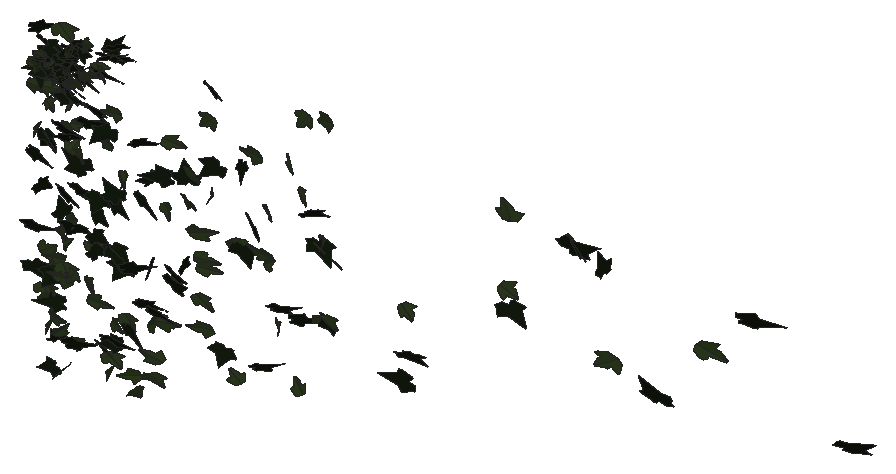
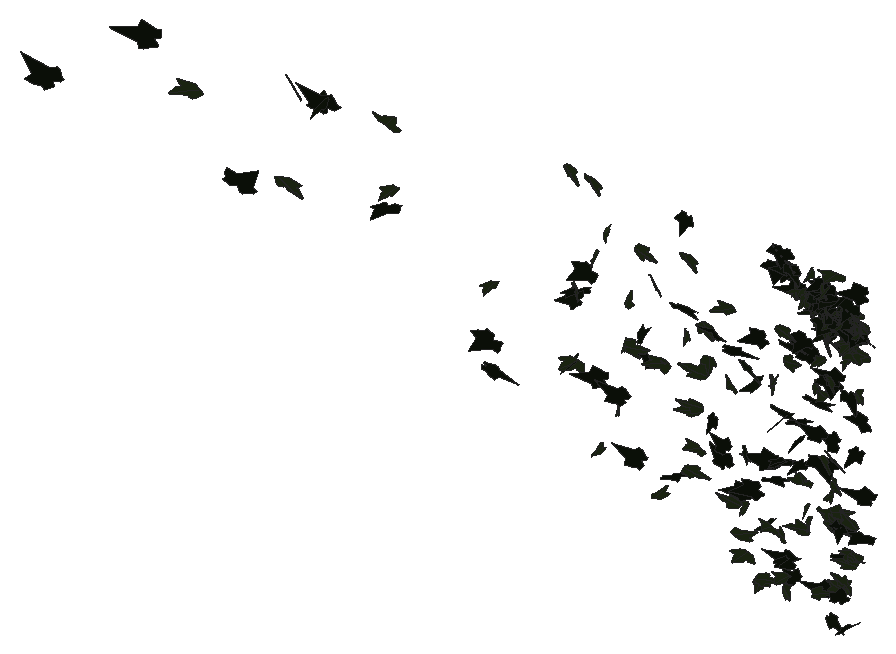
# SketchUp Ruby script. Lengths in millimetres.
U = 1.mm
M = Sketchup.active_model
def pt(a) = Geom::Point3d.new(a.map { |v| v * U })
def face(e, loops, mat)
  f = e.add_face(loops[0].map { |a| pt(a) })
  loops[1..].each { |l| e.add_face(l.map { |a| pt(a) }).erase! }
  f.material = f.back_material = mat if mat
  f
end
# faces: each face lists its corners as indices into pts; further lists are holes
def faces(e, pts, list, mat = nil) = list.each { |f| face(e, (f[0].is_a?(Array) ? f : [f]).map { |l| l.map { |i| pts[i] } }, mat) }
# xy, xz, yz: faces in a plane at the given z, y or x. An outline is a flat list of corners, or four numbers for a rectangle; further outlines are holes
def ring(l) = l.size == 4 ? [[l[0], l[1]], [l[2], l[1]], [l[2], l[3]], [l[0], l[3]]] : l.each_slice(2).to_a
def flat(e, list, mat, &to3) = list.each { |f| face(e, (f[0].is_a?(Array) ? f : [f]).map { |l| ring(l).map { |u, v| to3.(u, v) } }, mat) }
def xy(e, z, list, mat = nil) = flat(e, list, mat) { |x, y| [x, y, z] }
def xz(e, y, list, mat = nil) = flat(e, list, mat) { |x, z| [x, y, z] }
def yz(e, x, list, mat = nil) = flat(e, list, mat) { |y, z| [x, y, z] }
def lines(e, pts, list) = list.each { |a, b| e.add_line(pt(pts[a]), pt(pts[b])) }
# prism: a flat outline (further loops are holes) pulled along v
def prism(e, loops, v, mat = nil)
  f = face(e, loops, mat); d = Geom::Vector3d.new(v.map { |x| x * U })
  f.pushpull(f.normal.samedirection?(d) ? d.length : -d.length)
end
def box(e, o, s, mat = nil) = prism(e, [[o, [o[0] + s[0], o[1], o[2]], [o[0] + s[0], o[1] + s[1], o[2]], [o[0], o[1] + s[1], o[2]]]], [0, 0, s[2]], mat)
def at(x, y, z, deg = 0) = Geom::Transformation.translation(pt([x, y, z])) * Geom::Transformation.rotation(ORIGIN, Z_AXIS, deg.degrees)
def axes(o, x, y, z) = Geom::Transformation.new([*x, 0, *y, 0, *z, 0, *pt(o).to_a, 1])
def part(name) = M.definitions.add(name)
# library, detail: a bought-in or finely detailed component or shape, given as its bounding box
def library(name, o, s) = part(name).tap { |d| box(d.entities, o, s) }
def detail(e, o, s) = box(e.add_group.entities, o, s)
def put(e, d, t, mat = nil) = e.add_instance(d, t).tap { |i| i.material = mat if mat }
def group(e, t, mat = nil) = e.add_group.tap { |g| g.transformation = t; g.material = mat if mat }.entities
root = M.entities
M.materials.add("efeu1").color = [18, 25, 13]
M.materials.add("efeu2").color = [43, 57, 29]
c1 = part("ivyleaf_9")
p = [[39.1,54.8,31.7],[34.5,51.8,30.2],[-5.3,25.2,17.3],[-17.9,28.3,20.9],[-21.6,21.7,17],[-20.2,4.3,5.3],
  [-22.9,-0.3,2.5],[-17.1,-4,-0.6],[-2,-2.1,-1.2],[-0.7,-15.4,-10.1],[16.6,-22.3,-16.7],[21.1,-15.1,-12.5],
  [32.7,-10.7,-11],[46.1,-1.8,-6.6],[30.8,11.2,3.8]]
faces(c1.entities,p,[[0,1,2,3,4,5,6,7,8,9,10,11,12,13,14]],"efeu1")
c2 = part("ivyleaf_10")
p = [[0,12.8,-0.8],[-1.5,51.3,-10.9],[-4.9,51,-11.6],[-13.6,26.5,-7.3],[-13.2,15.9,-4.6],[-21.1,19.3,-7.2],
  [-29.5,16.3,-8.3],[-29.2,8.3,-6.2],[-19.7,-9.8,0.5],[-7.6,-13,4],[1,-12.2,5.8],[-0.4,51.1,-11.1],
  [-1.5,51.1,-10.9],[1,-12.4,5.9],[16.9,-12.4,3.5],[35.1,9.1,-5.1],[35,12.9,-6.1],[20.5,16.4,-4.9],
  [15.8,15,-3.8],[15.3,27.6,-7.1],[12.8,31.3,-7.8]]
faces(c2.entities,p,[[0,1,2,3,4,5,6,7,8,9,10],[11,12,0,13,14,15,16,17,18,19,20]],"efeu2")
put(root,c1,axes([2770.4,996,647.1],[-0.43445,-0.41546,-0.67356],[0.58698,0.59889,-0.47393],[1.38708,-0.38357,-0.01041]))
put(root,c1,axes([2810.1,994.4,1431.9],[-1.27919,0.3991,0.09668],[-0.21391,-0.00043,-0.77958],[-0.75169,-0.67905,0.05732]))
put(root,c1,axes([2754.7,988,793.5],[0.65605,-0.1407,0.72585],[1.38247,-0.08487,-0.36142],[0.26236,0.79905,0.08942]))
put(root,c2,axes([2790.1,1023.7,1355.9],[1.07633,0.46383,-0.26625],[-0.4274,-0.14573,-0.73088],[-0.92378,0.60785,0.02794]))
put(root,c2,axes([2787.5,994.3,1427.6],[0.14869,0.78127,-0.03035],[-0.07273,-0.02665,-0.78437],[-1.48625,0.07947,0.03535]))
put(root,c2,axes([2792.4,997.3,1191.2],[0.28219,-0.75376,0.3272],[0.17611,-0.31505,-0.76771],[1.55394,0.17259,0.02758]))
put(root,c2,axes([2766.3,990.4,1346.9],[-0.16001,-0.05129,-0.78981],[1.38192,-0.32107,-0.05644],[-0.59945,-0.72649,0.0807]))
put(root,c1,axes([2795.2,996.2,965.3],[0.00384,-0.03525,-0.90722],[-0.71675,0.82546,-0.03291],[1.57226,0.37639,-0.01279]))
put(root,c2,axes([2788.9,993.1,1443.8],[0.95422,0.59568,0.11552],[0.13095,0.09307,-0.77857],[-1.14738,0.50602,0.00721]))
put(root,c1,axes([2792.6,992.2,1426.2],[1.13022,0.51418,-0.05023],[-0.05686,-0.04222,-0.78542],[-0.9816,0.59447,-0.01234]))
put(root,c1,axes([2767.1,988.9,1088.7],[0.30092,0.00107,-0.85529],[1.60853,0.13322,0.15641],[0.24969,-0.85952,0.02318]))
put(root,c2,axes([2793,983.8,1457.4],[-1.08334,-0.41986,-0.41689],[0.75174,0.16106,-0.70152],[0.83841,-0.68693,0.09033]))
put(root,c2,axes([2807,987.4,1445.8],[0.11013,-0.79891,-0.00714],[-0.00685,0.00689,-0.801],[1.52054,0.05789,-0.00309]))
put(root,c1,axes([2781.9,983.3,1575.3],[0.73988,0.19969,0.83467],[1.34298,0.44717,-0.43565],[-0.92968,0.80489,0.03495]))
put(root,c2,axes([2802.5,994.8,1447.7],[1.4992,0.02043,-0.01835],[-0.03497,0.00059,-0.78799],[-0.03885,0.78794,0.00107]))
put(root,c2,axes([2802.8,991.4,1449.2],[-1.33687,-0.27071,-0.23913],[0.49196,-0.01151,-0.74628],[0.48015,-0.74193,0.09883]))
put(root,c1,axes([2805.9,1006.1,1383.4],[-0.66525,-0.66942,0.19408],[0.26549,-0.27992,-0.71426],[1.29967,-0.28547,0.24525]))
put(root,c2,axes([2819,988.8,1464.8],[0.9697,-0.57099,-0.2545],[-0.29405,0.20312,-0.76504],[1.15286,0.53209,0.01893]))
put(root,c2,axes([2814.6,999.8,1395.3],[1.01038,-0.57852,-0.03027],[0.03136,0.05612,-0.78359],[1.10209,0.52878,0.05005]))
put(root,c2,axes([2840.3,1003.5,561.3],[0.2043,-0.03721,-0.82761],[-1.0817,0.60385,-0.10087],[1.14712,0.57604,0.05228]))
put(root,c2,axes([2792.4,1024.7,693.5],[1.22553,-0.29947,-0.58382],[0.99236,-0.26303,0.71002],[-0.75808,-0.82844,-0.01438]))
put(root,c2,axes([2820.9,992.6,1452.9],[0.60866,-0.72349,0.08485],[0.04614,-0.08205,-0.79094],[1.38561,0.32054,-0.01093]))
put(root,c1,axes([2840,989.6,1489.5],[-1.40065,0.33106,-0.02115],[0.03029,-0.01618,-0.80694],[-0.63064,-0.73607,0.00822]))
put(root,c2,axes([2817,997.9,1352.8],[-0.27329,0.77613,-0.04261],[0.00584,-0.04276,-0.78928],[-1.47934,-0.14355,0.00475]))
put(root,c2,axes([2804,1003.3,564.9],[1.19157,0.40959,0.3594],[0.57515,0.19454,-0.74816],[-0.86298,0.6952,-0.00239]))
put(root,c2,axes([2816.8,1017.1,1364.9],[-0.19462,0.77125,-0.0598],[0.06221,-0.05596,-0.7776],[-1.47094,-0.10441,-0.02497]))
put(root,c1,axes([2814,983.9,1466.8],[0.99592,0.48237,0.35709],[0.27901,0.35668,-0.69664],[-1.10763,0.52356,0.1456]))
put(root,c1,axes([2816.5,999.2,1529.1],[1.57904,-0.09375,-0.44782],[-0.83876,0.08533,-0.83438],[0.23389,0.93895,0.03111]))
put(root,c2,axes([2828.6,987.4,1491.6],[-0.86769,-0.66819,0.06412],[0.0778,-0.105,-0.80359],[1.27517,-0.44826,0.09265]))
put(root,c2,axes([2837,986.9,1489.5],[-1.3935,-0.32756,0.14451],[-0.2277,-0.0862,-0.80158],[0.6422,-0.74132,0.02935]))
put(root,c1,axes([2843.3,981.9,1165.2],[0.81962,-0.00474,-0.7673],[-1.45921,-0.03747,-0.43009],[-0.05779,0.87909,-0.02247]))
put(root,c1,axes([2830.5,994.4,1463.7],[-0.95004,-0.51061,-0.35288],[0.50207,0.23537,-0.71375],[1.06928,-0.56419,0.0216]))
put(root,c2,axes([2816.9,998.8,519.8],[-0.33431,-0.28464,0.76462],[0.89721,0.60295,0.33276],[-1.26733,0.50194,0.03388]))
put(root,c2,axes([2837.4,1005.3,434.8],[0.27791,-0.75395,0.32438],[0.17599,-0.31227,-0.76741],[1.55214,0.1704,0.02893]))
put(root,c1,axes([2823.8,990.7,1177.3],[0.36354,-0.8108,-0.17875],[-0.05325,0.17702,-0.83289],[1.57927,0.19261,0.01306]))
put(root,c1,axes([2846.4,1015,264.3],[0.15599,-0.58274,-0.5782],[0.25317,-0.56396,0.58725],[-1.54171,-0.15157,0.03793]))
put(root,c2,axes([2832.3,998.5,1365.3],[0.44168,0.64421,0.40094],[0.19527,0.38878,-0.68406],[-1.43086,0.25191,0.03041]))
put(root,c2,axes([2823.6,996.5,1407.2],[1.05938,-0.13923,0.53905],[1.00082,-0.11887,-0.57371],[0.34801,0.76569,0.00895]))
put(root,c2,axes([2841.7,986,1303.8],[0.04143,0.74231,0.25477],[-0.04327,0.25536,-0.74208],[-1.49303,0.0132,0.02858]))
put(root,c1,axes([2870.4,994.8,1425.3],[-1.28735,-0.14968,0.385],[-0.70842,-0.09942,-0.69262],[0.34087,-0.77193,0.01455]))
put(root,c1,axes([2867.5,988.5,1465.4],[-0.68853,0.69928,0.12269],[-0.07586,0.11747,-0.7871],[-1.34906,-0.3635,-0.01835]))
put(root,c1,axes([2881.3,1002.5,525.4],[-0.94111,-0.09724,0.67365],[-1.24284,-0.16694,-0.50345],[0.36516,-0.81881,0.02264]))
put(root,c1,axes([2865.8,996.3,1437.2],[0.48306,0.72266,-0.20686],[-0.42958,-0.13499,-0.74852],[-1.36459,0.29832,0.16241]))
put(root,c2,axes([2851.7,990.1,684.9],[0.65418,-0.75002,0.12988],[-0.10386,0.11786,0.82503],[-1.44496,-0.34803,-0.0005]))
put(root,c1,axes([2859.7,1016,377],[0.64878,0.25534,0.67418],[-1.04133,-0.39395,0.42586],[0.89339,-0.64462,0.00679]))
put(root,c1,axes([2868.1,995.8,638.5],[-1.30956,-0.47,0.07682],[-0.11134,-0.05055,-0.83323],[0.8995,-0.69051,0.00871]))
put(root,c2,axes([2863.4,993.1,1481.9],[1.11389,0.44455,-0.31867],[-0.54814,-0.1463,-0.73305],[-0.88499,0.65015,0.05294]))
put(root,c2,axes([2835.7,1021.1,449.4],[-0.4908,0.06992,0.74698],[1.38175,-0.17588,0.2671],[0.35999,0.77042,-0.00682]))
put(root,c1,axes([2870.2,988.2,1349.7],[-0.6251,0.58445,-0.4236],[0.41108,-0.36448,-0.67037],[-1.31081,-0.39302,-0.00822]))
put(root,c2,axes([2885.4,1001.1,701.7],[-0.30057,-0.04586,-0.80992],[-1.3275,-0.4136,0.15943],[-0.78827,0.71403,0.04033]))
put(root,c1,axes([2899.3,984.6,1442.2],[-0.30189,-0.08005,-0.94213],[-1.6694,-0.3442,0.17693],[-0.67184,0.89123,-0.01629]))
put(root,c2,axes([2847,975.8,1371.7],[-0.23971,-0.28137,-0.73434],[1.12844,0.45457,-0.27587],[0.98318,-0.59033,0.13758]))
put(root,c1,axes([2859,972.6,1533.9],[0.527,-0.24019,-0.80036],[-0.47252,0.78143,-0.32041],[1.51854,0.32652,0.17806]))
put(root,c1,axes([2873.2,997.8,655.8],[1.12675,-0.06235,-0.60081],[-1.14058,0.0446,-0.59516],[0.1438,0.84231,-0.01296]))
put(root,c2,axes([2865.2,997.4,1431.5],[-0.10373,0.76435,0.1995],[0.01486,0.20049,-0.766],[-1.50338,-0.05076,-0.02134]))
put(root,c1,axes([2903.8,991.3,1440.9],[-0.91114,0.4472,0.46501],[-0.65885,0.31057,-0.65508],[-1.03612,-0.59074,0.00763]))
put(root,c2,axes([2902.7,992.9,806],[-0.27567,0.11536,0.83732],[-1.34565,0.44895,-0.18417],[-0.88144,-0.72148,0.01928]))
put(root,c2,axes([2874.4,997.8,409.8],[-0.32368,-0.65855,0.49115],[0.18926,0.48137,0.67987],[-1.55203,0.19604,-0.01953]))
put(root,c2,axes([2919.6,985.8,643.1],[0.49505,-0.05093,-0.9672],[-1.78641,0.23369,-0.26474],[0.45453,0.97392,0.01294]))
put(root,c1,axes([2912.1,985.2,893.5],[-1.25258,0.3832,-0.52809],[-0.87011,0.26432,0.76157],[0.88597,0.80135,0.00133]))
put(root,c1,axes([2872.9,992.3,1488.5],[0.72176,-0.70472,-0.05999],[0.05625,0.0838,-0.79759],[1.3449,0.37469,0.06555]))
put(root,c1,axes([2906.6,994,1455.8],[-0.17798,0.73235,-0.30272],[-0.05028,-0.30753,-0.73583],[-1.50736,-0.07621,0.06029]))
put(root,c1,axes([2888.6,992.2,1397.8],[0.86753,-0.39345,-0.52624],[-0.73427,0.35818,-0.60197],[1.01225,0.59701,0.01435]))
put(root,c1,axes([2906.1,1002,284.6],[-0.64566,0.575,-0.45103],[0.39578,-0.40075,-0.66731],[-1.33334,-0.3974,0.02033]))
put(root,c2,axes([2911.4,1010.1,1217.6],[0.91062,-0.56999,-0.45075],[-0.41121,0.4037,-0.73983],[1.32048,0.51879,0.08046]))
put(root,c2,axes([2904.7,994.1,1412.8],[-1.08474,-0.52951,-0.176],[0.33485,0.06821,-0.77498],[1.00779,-0.5926,0.06806]))
put(root,c2,axes([2903.5,1000.6,764.7],[0.03441,-0.02662,-0.82961],[0.33347,0.81123,-0.02221],[1.54413,-0.1746,0.02328]))
put(root,c1,axes([2931.1,982.2,1349.2],[-0.77924,0.54734,0.41119],[-0.44009,0.34039,-0.68335],[-1.22634,-0.46995,-0.01605]))
put(root,c1,axes([2916.9,989.4,1197.8],[0.75091,0.673,-0.20865],[-0.24643,-0.1658,-0.77966],[-1.31815,0.41439,0.0269]))
put(root,c1,axes([2884.1,995.5,1215.7],[0.72504,-0.32428,0.67991],[1.09943,-0.36322,-0.49691],[0.9201,0.68954,0.058]))
put(root,c1,axes([2885.9,998.7,970.1],[0.75972,-0.04846,-0.86177],[1.62285,-0.12509,0.40201],[-0.25473,-0.94146,-0.00905]))
put(root,c2,axes([2900.8,985.4,1615],[1.31033,0.51649,0.42703],[0.67541,0.23836,-0.86045],[-1.08194,0.77431,-0.01996]))
put(root,c2,axes([2908.1,987.8,686.7],[1.15339,0.53614,0.23703],[0.32321,0.16573,-0.80907],[-1.06782,0.62927,0.01114]))
put(root,c2,axes([2937,995.8,1416.5],[-1.68835,0.24227,0.29678],[-0.54565,0.07669,-0.9196],[-0.48362,-0.93229,0.00147]))
put(root,c2,axes([2928.9,992.1,1467.4],[0.16721,-0.79549,0.02743],[0.02046,-0.02641,-0.80029],[1.51474,0.08817,0.00778]))
put(root,c2,axes([2944.3,1033.2,379.9],[0.05367,0.00844,-0.81112],[-1.11624,-0.56045,-0.02622],[-1.06646,0.58703,-0.01338]))
put(root,c1,axes([2940.2,991.2,1477.2],[0.61089,0.53495,-0.50611],[-0.5153,-0.4277,-0.62379],[-1.30339,0.41982,0.00941]))
put(root,c1,axes([2925.7,991.4,1420],[1.31334,0.41373,-0.01781],[-0.26393,0.19826,-0.76756],[-0.74264,0.66122,0.24129]))
put(root,c2,axes([2946.6,992.4,879.6],[0.55312,-0.41594,-0.70162],[-0.68614,0.60261,-0.50658],[1.39247,0.46216,0.02908]))
put(root,c1,axes([2904.7,992.8,1400.5],[1.09123,-0.49432,0.26465],[0.43205,-0.14146,-0.75604],[0.97577,0.61545,0.03879]))
put(root,c2,axes([2936.3,989.5,1428.3],[-0.04089,-0.80655,-0.001],[0.00826,0.00089,-0.80682],[1.53501,-0.02149,0.00431]))
put(root,c2,axes([2926.3,1005.4,1140.1],[0.58091,0.55657,-0.56846],[0.56212,0.48607,0.63449],[1.4059,-0.42432,-0.01881]))
put(root,c2,axes([2939.5,986.4,1335.9],[0.70165,-0.7287,-0.08806],[-0.06859,0.08045,-0.81664],[1.39526,0.3704,0.00414]))
put(root,c1,axes([2935.7,971.7,1513.5],[0.97736,0.57418,0.22881],[0.05682,0.2741,-0.75481],[-1.17498,0.49086,0.15383]))
put(root,c2,axes([2934.1,980.1,1538.5],[0.04214,-0.40999,-0.7123],[0.50776,0.67755,-0.3817],[1.47946,-0.22086,0.15129]))
put(root,c1,axes([2922.1,982.8,1505.3],[0.01935,0.00045,0.82155],[1.47895,0.26663,-0.00976],[-0.50743,0.77715,0.00287]))
put(root,c2,axes([2949.3,984.7,1552],[-0.05168,-0.80702,-0.12925],[0.01292,0.1291,-0.80747],[1.55544,-0.02788,0.00242]))
put(root,c2,axes([2946.4,987.6,674],[1.42499,-0.40509,-0.04828],[-0.08043,0.02335,-0.85129],[0.77224,0.74992,0.00043]))
put(root,c1,axes([2960.3,980.8,867.2],[0.99062,0.48408,-0.60741],[-0.88871,-0.38927,-0.71037],[-1.18126,0.69881,0.02506]))
put(root,c1,axes([2920.8,1003,381],[0.46671,-0.05088,0.81395],[1.55206,0.02395,-0.24419],[-0.0158,0.84975,0.05562]))
put(root,c1,axes([2942.3,980.4,1556.4],[1.38715,0.34667,-0.05581],[-0.13455,0.01892,-0.8057],[-0.65459,0.73074,0.04734]))
put(root,c1,axes([2937.8,976.1,1370.8],[1.3112,-0.28627,-0.37646],[-0.39421,0.41535,-0.69491],[0.80918,0.66622,0.27147]))
put(root,c1,axes([2992.4,992.7,1092.9],[-1.68059,-0.16496,-0.3684],[-0.69032,-0.06456,0.8983],[-0.3371,0.95462,-0.00291]))
put(root,c1,axes([2954.9,981.6,1564.1],[0.17143,0.03024,-0.81627],[-0.26384,0.80987,0.0147],[1.53204,0.13609,0.09387]))
put(root,c2,axes([2959.6,984.7,1260.4],[0.04818,0.28221,0.75815],[0.03017,0.7582,-0.28276],[-1.53934,0.02369,0.01819]))
put(root,c2,axes([2995.5,974.7,1147],[-0.21904,0.06058,0.89347],[-1.38775,0.51661,-0.12895],[-0.98943,-0.738,-0.01693]))
put(root,c1,axes([2953.5,996.2,1484.2],[1.13573,-0.53668,-0.01954],[-0.04151,0.00497,-0.8025],[1.02124,0.59705,-0.01089]))
put(root,c1,axes([2944.7,1015.5,982.1],[0.36546,-0.19658,0.77799],[1.2229,-0.44151,-0.27015],[0.9148,0.66874,0.05033]))
put(root,c1,axes([2989.3,973.9,1479],[0.08173,0.79783,0.13048],[-0.04538,0.13186,-0.79841],[-1.53794,0.03851,0.03049]))
put(root,c2,axes([2978.9,989.3,1456.6],[-0.34019,0.7869,0.03925],[-0.02509,0.03725,-0.80694],[-1.49929,-0.17917,0.0046]))
put(root,c2,axes([2988.8,1011.7,642.4],[-0.71493,0.62219,0.36467],[-0.40167,0.29833,-0.72641],[-1.31247,-0.43022,0.02367]))
put(root,c1,axes([2987.5,975.5,1559.6],[0.79675,-0.09963,-0.78482],[-0.98196,0.63873,-0.3563],[1.14139,0.61905,0.24132]))
put(root,c1,axes([2971.4,987.7,1451],[1.02507,-0.60321,-0.07073],[0.2358,0.20168,-0.77649],[1.13158,0.50441,0.22588]))
put(root,c2,axes([3013.2,986.8,1472.5],[-0.2206,-0.80635,0.00121],[0.03825,-0.00411,-0.81438],[1.53418,-0.11584,0.02048]))
put(root,c2,axes([3006.2,981.4,1588],[0.05012,-0.46906,-0.67824],[0.37558,0.66245,-0.45048],[1.52384,-0.14785,0.13334]))
put(root,c1,axes([2993.9,993.1,1270.2],[1.34327,0.31997,-0.30043],[0.40448,0.24863,0.76407],[0.73087,-0.72566,0.12931]))
put(root,c2,axes([3025.1,981.7,664.1],[-0.52941,0.77347,0.24377],[-0.17623,0.22573,-0.8219],[-1.53335,-0.29299,0.0103]))
put(root,c2,axes([3018.5,1015.6,778.3],[1.50704,0.19229,-0.11739],[0.1935,0.07781,0.81326],[0.38262,-0.79671,0.05109]))
put(root,c1,axes([3017.3,1004.6,1334],[1.48059,0.04309,-0.26893],[-0.51339,0.00954,-0.77879],[-0.07156,0.82306,0.0231]))
put(root,c2,axes([3025.9,984.9,1481.9],[-0.36774,-0.5596,-0.56445],[0.42256,0.51977,-0.5913],[1.45251,-0.29289,0.02912]))
put(root,c1,axes([3053.4,991.6,782.2],[-1.22756,0.3125,-0.45456],[-0.79646,0.17843,0.71647],[0.68396,0.76864,0.01848]))
put(root,c1,axes([3027.7,1003.4,846.5],[0.21544,-0.31602,-0.74694],[-0.32726,0.72768,-0.33393],[1.50848,0.203,0.03423]))
put(root,c1,axes([3041.4,1000.4,933],[0.49346,-0.45785,-0.63289],[-0.58879,0.55213,-0.52617],[1.3651,0.40365,0.00183]))
put(root,c2,axes([3044.2,1000.2,1508.6],[0.77852,0.69555,0.05472],[0.05515,0.04644,-0.80692],[-1.32671,0.41008,-0.00143]))
put(root,c1,axes([3054.8,1002.8,999.1],[-0.93467,-0.66212,0.06401],[-0.05909,-0.05666,-0.82433],[1.26464,-0.49201,0.00879]))
put(root,c2,axes([3024.5,1001.7,587.5],[0.20592,0.05044,0.83793],[1.39993,0.40139,-0.11914],[-0.76981,0.74344,0.00748]))
put(root,c1,axes([3040.8,1028.9,398],[0.37911,-0.46664,0.64707],[0.51526,-0.58781,-0.50725],[1.42822,0.33593,0.01124]))
put(root,c2,axes([3093.6,1002,1217.2],[-0.38138,0.20317,-0.7828],[-1.17995,0.47927,0.2831],[0.98836,0.65057,0.03591]))
put(root,c2,axes([3072.2,981.8,1510.2],[0.18022,-0.76625,-0.28768],[0.01745,0.29058,-0.77094],[1.55762,0.0854,0.04192]))
put(root,c2,axes([3071.7,981.3,1506.7],[-0.46716,0.78445,0.04881],[-0.00514,0.05029,-0.82187],[-1.49585,-0.24516,-0.01242]))
put(root,c1,axes([3094.7,997.8,1280.2],[-1.85861,-0.05472,-0.15829],[0.30077,0.00906,-0.9781],[0.10557,-0.98928,-0.00021]))
put(root,c1,axes([3096.5,982.3,1574.8],[-0.25312,0.81127,0.00535],[-0.01081,0.00449,-0.82208],[-1.544,-0.13303,0.00488]))
put(root,c1,axes([3052.4,982.9,1498.2],[1.24097,-0.24081,0.43804],[0.85177,-0.03946,-0.68788],[0.42376,0.78453,0.09986]))
put(root,c2,axes([3113.9,1016.5,1340.3],[0.63036,-0.14022,-0.75629],[-1.2836,0.34297,-0.35895],[0.70386,0.75104,0.02271]))
put(root,c2,axes([3090.7,1019.8,336.5],[0.24382,-0.82101,0.27076],[0.14043,-0.26233,-0.83037],[1.63932,0.14458,0.03086]))
put(root,c1,axes([3113.5,1025.9,436.1],[-0.50475,-0.21482,0.76067],[-1.14841,-0.46324,-0.3412],[0.97169,-0.65907,-0.00812]))
put(root,c1,axes([3123.3,1012,1015],[-1.58707,0.0537,-0.27122],[-0.51631,0.0075,0.83557],[0.1016,0.87686,0.00946]))
put(root,c2,axes([3083.5,1017.5,387],[1.13677,0.41037,0.48709],[0.71814,0.30997,-0.72385],[-0.97655,0.70564,0.03469]))
put(root,c1,axes([3101,982.8,1576.8],[1.30375,0.42401,-0.16594],[-0.43315,0.05921,-0.78822],[-0.75056,0.70235,0.16663]))
put(root,c1,axes([3087.4,980.4,1560.6],[0.85885,0.02852,0.69238],[1.03634,0.49644,-0.37535],[-0.81571,0.66074,0.25213]))
put(root,c1,axes([3074.4,1009.2,450.4],[0.92182,0.23023,-0.68763],[1.17172,0.30638,0.53623],[0.72923,-0.78331,0.00763]))
put(root,c1,axes([3104,992.4,1590.8],[-0.65577,0.83228,0.41351],[0.29607,-0.38314,0.90078],[1.74377,0.37804,0.00256]))
put(root,c1,axes([3106.7,1013.5,992.6],[0.73998,-0.57137,-0.53863],[-0.45849,0.48526,-0.68865],[1.42238,0.45367,0.05823]))
put(root,c1,axes([3112.8,1003.6,825.7],[-0.06965,-0.55673,-0.61185],[0.28207,0.59813,-0.55311],[1.54892,-0.13396,0.07321]))
put(root,c1,axes([3121.4,1003.1,812.3],[-0.1699,-0.80801,-0.15941],[0.03612,0.15828,-0.81292],[1.56702,-0.09125,0.00146]))
put(root,c1,axes([3135.5,978.5,1625.1],[0.72816,0.73048,-0.09898],[-0.08993,-0.08698,-0.82461],[-1.40007,0.3855,0.00149]))
put(root,c1,axes([3136.8,1002.5,1571.7],[1.02835,0.60153,-0.1539],[-0.29284,-0.06792,-0.80572],[-1.14485,0.5577,0.06786]))
put(root,c1,axes([3144.1,1025.6,753.9],[-1.20425,-0.55748,0.05586],[-0.07543,-0.03952,-0.84329],[1.06364,-0.63398,0.00344]))
put(root,c2,axes([3113,1005.2,528.1],[0.17904,-0.03316,0.82359],[1.3735,-0.39717,-0.09842],[0.7579,0.72761,-0.01619]))
put(root,c2,axes([3151.9,996,1123.5],[-0.14135,0.82558,-0.12962],[0.02674,-0.12888,-0.82891],[-1.59028,-0.07555,-0.00242]))
put(root,c2,axes([3172.3,992.6,1118.6],[0.33972,-0.81261,-0.54024],[-0.09674,0.54071,-0.83012],[1.85463,0.17706,0.05566]))
put(root,c2,axes([3192.8,1024.4,346],[0.31032,0.08602,-0.82421],[-1.34793,-0.42167,-0.18411],[-0.81885,0.72671,-0.00927]))
put(root,c2,axes([3153.6,1020.2,558.8],[1.23937,-0.03728,0.52916],[1.00113,-0.06297,-0.65177],[0.13056,0.83673,-0.02548]))
put(root,c1,axes([3185,989.9,544],[0.74659,-0.79365,-0.08846],[-0.0618,0.08262,-0.88527],[1.51857,0.39355,0.00747]))
put(root,c1,axes([3191.4,975.3,779.4],[0.62038,0.03667,0.9143],[1.61848,0.34617,-0.31707],[-0.64291,0.90685,0.08406]))
put(root,c2,axes([3222.4,986.9,314.7],[-0.59807,-0.69836,-0.44569],[0.37011,0.40118,-0.76573],[1.53268,-0.36938,0.01099]))
put(root,c1,axes([3206.2,999.3,1265.7],[0.93421,0.31504,0.62351],[0.97594,0.35502,-0.58307],[-0.9029,0.7097,0.01489]))
put(root,c1,axes([3275.9,1009.4,1147.4],[-0.88156,0.72519,0.08071],[-0.09193,0.06491,-0.86048],[-1.38566,-0.46568,0.00574]))
put(root,c1,axes([3235.9,986.7,1074.4],[1.1087,-0.7949,-0.16081],[-0.18107,0.12965,-0.98551],[1.53285,0.59026,-0.0001]))
put(root,c1,axes([3239.1,988.9,660.3],[1.34981,0.1518,0.48928],[0.90959,0.10484,-0.72529],[-0.3511,0.85523,0.00207]))
put(root,c1,axes([3266.4,1021.6,813.8],[-0.69733,0.30158,-0.71827],[1.07177,-0.44591,-0.47449],[-1.02442,-0.6718,-0.00749]))
put(root,c2,axes([3281.2,994.6,581.9],[-0.033,0.16119,0.86373],[-0.50514,0.82258,-0.15884],[-1.59411,-0.264,0.03245]))
put(root,c2,axes([3312.7,992.2,460.8],[0.74306,0.36257,0.70909],[-1.02981,-0.45868,0.53246],[1.11215,-0.66697,0.01928]))
put(root,c2,axes([3291,990.3,392.9],[-1.40319,-0.21023,-0.44186],[0.8176,0.10451,-0.76652],[0.44591,-0.85317,0.01499]))
put(root,c1,axes([3281.1,997,638.3],[1.30001,-0.26172,0.43688],[0.77499,-0.15828,-0.73149],[0.5821,0.79523,-0.0018]))
put(root,c1,axes([3346.5,1005.3,1176],[-1.20795,-0.02,0.59964],[-1.14107,-0.01162,-0.63499],[0.04286,-0.87308,-0.00529]))
put(root,c2,axes([3309.3,1017.8,596.8],[0.39142,-0.11772,-0.82357],[1.55541,-0.1301,0.22269],[-0.29616,-0.83884,0.08104]))
put(root,c2,axes([3326.2,1018,1053.9],[1.00179,-0.38449,0.56942],[0.91741,-0.3045,-0.6512],[0.93183,0.71315,0.02895]))
put(root,c1,axes([3344.4,1032.9,745.2],[-0.14014,-0.09714,0.93771],[0.8731,-0.82538,-0.04948],[1.56744,0.45107,0.1114]))
put(root,c1,axes([3351.9,1022.8,796],[0.24619,-0.34532,0.7892],[0.67451,-0.70605,-0.36703],[1.49432,0.37559,0.03565]))
put(root,c2,axes([3354.6,994.5,1329.3],[0.43808,0.28887,0.79062],[0.90357,0.63227,-0.36924],[-1.32286,0.52753,0.00961]))
put(root,c2,axes([3427.9,1013.6,1110.6],[-1.29431,0.42949,0.3523],[-0.55,0.20207,-0.80419],[-0.90291,-0.73877,-0.01515]))
put(root,c1,axes([3425.8,989.5,873.9],[-0.02742,0.02755,-0.86653],[-0.99548,0.69088,0.03067],[1.31589,0.52323,0.00514]))
put(root,c1,axes([3442.6,997,1203.4],[-1.68994,0.24223,0.00977],[0.01043,-0.01704,0.92027],[0.46127,0.88784,0.015]))
put(root,c2,axes([3462.5,998.4,1224.8],[-1.06067,0.18337,0.66664],[-1.23124,0.1638,-0.58589],[-0.46426,-0.85333,0.03079]))
put(root,c2,axes([3518.3,1005.9,648.2],[0.48066,0.01161,-0.84553],[-1.6093,0.01163,-0.25241],[0.01489,0.88237,0.01445]))
put(root,c2,axes([3473.7,1014.7,750.8],[1.04148,0.0551,0.68695],[1.2969,0.08767,-0.54987],[-0.19577,0.87388,0.01185]))
put(root,c2,axes([3486.2,979.5,1021.7],[-0.69591,-0.34592,0.89352],[1.26615,0.5966,0.50321],[-1.31232,0.75905,0.01168]))
put(root,c2,axes([3480.2,1010.6,909.5],[0.01841,-0.03559,-0.88536],[1.68604,-0.01726,0.01037],[-0.03362,-0.88524,0.0354]))
put(root,c2,axes([3532.2,1002.7,1470.3],[1.3346,-0.45029,-0.44963],[-0.66563,0.28624,-0.83212],[1.01176,0.78229,0.04566]))
put(root,c2,axes([3501,999.2,882.4],[0.17274,0.07216,0.87669],[1.05235,0.68078,-0.11328],[-1.30206,0.55979,0.02476]))
put(root,c2,axes([3533.8,1004.8,1174.7],[0.04112,-0.54033,-0.71714],[-0.00467,0.71731,-0.54053],[1.70891,0.01496,0.01578]))
put(root,c1,axes([3547.5,1025.5,1284.1],[-1.66905,-0.16565,0.00713],[-0.01286,-0.00261,-0.89248],[0.3153,-0.87699,0.00131]))
put(root,c1,axes([3548.1,983.3,1609.6],[1.27284,-0.11344,-0.57789],[-1.05829,0.16634,-0.67618],[0.36912,0.86808,0.05405]))
put(root,c1,axes([3597.8,1003.1,596],[-0.85107,-0.7709,0.06351],[-0.06105,-0.05481,-0.89121],[1.47089,-0.44833,-0.00024]))
put(root,c2,axes([3655.7,1002.8,497],[0.39362,0.83198,0.2688],[-0.15095,-0.25722,0.85718],[1.65714,-0.22105,0.01424]))
put(root,c2,axes([3634.2,1009.7,1025.6],[-0.95979,-0.06075,-0.75277],[1.41652,0.11352,-0.50778],[0.24375,-0.89895,-0.01325]))
put(root,c1,axes([3661.2,1019.8,1333.3],[-0.86611,0.08926,-0.77845],[1.37001,-0.30794,-0.45613],[-0.58902,-0.8475,0.08375]))
put(root,c1,axes([3674.7,1006.6,1022.8],[-1.01791,-0.33666,-0.65792],[1.09073,0.32386,-0.63161],[0.88811,-0.78361,0.02162]))
put(root,c2,axes([3749.8,984.8,1412.4],[0.29905,-0.0854,-0.9413],[-1.47747,0.53265,-0.17791],[1.0261,0.79184,0.01816]))
put(root,c1,axes([3734.2,1006.3,1088.5],[-0.0427,-0.66644,0.68137],[0.03865,0.68107,0.66681],[-1.81354,0.03021,-0.00183]))
put(root,c2,axes([3783.4,995.8,1027.3],[-0.57742,0.1796,-0.85444],[-1.5758,0.22789,0.3419],[0.52737,0.8776,0.08607]))
put(root,c1,axes([3754.4,979.4,593],[1.03185,0.73882,-0.28624],[0.31761,0.23258,0.9164],[1.47414,-0.56726,0.00292]))
put(root,c2,axes([3794.7,995.1,1192.6],[-1.08247,0.70129,0.19131],[0.20874,-0.15734,0.90284],[1.36763,0.57908,0.01362]))
put(root,c2,axes([3809.3,968.2,1019.5],[-0.09682,0.15909,0.89723],[-0.44059,0.86688,-0.16683],[-1.67734,-0.23689,-0.00797]))
put(root,c2,axes([3840.6,985.4,775.2],[0.25835,-0.20911,-0.8898],[-0.10626,0.89598,-0.21909],[1.73636,0.08595,0.11898]))
put(root,c1,axes([3808.9,1009.9,828.7],[1.28766,0.5524,-0.30883],[0.45961,0.19253,0.87344],[1.11334,-0.71838,-0.00339]))
put(root,c2,axes([3907.8,973.1,1419.6],[-0.24582,0.63905,-0.68012],[-0.37944,0.65186,0.65036],[1.73516,0.23308,0.04587]))
put(root,c2,axes([3934.7,988.5,559.4],[0.15194,0.92735,-0.03059],[-0.04068,0.03253,0.93047],[1.76543,-0.07906,0.02407]))
put(root,c2,axes([3938.5,988.4,1332.1],[-0.49124,0.89152,0.14434],[-0.09043,0.1365,-0.92811],[-1.71646,-0.26234,0.00759]))
put(root,c2,axes([3948.5,1002.7,1625.5],[1.47641,-0.56855,-0.25553],[-0.3773,0.16173,-0.96171],[1.12474,0.80058,0.01282]))
put(root,c1,axes([3926.9,973.2,841],[0.82318,0.10417,0.82238],[1.50816,0.22035,-0.44468],[-0.46314,0.90268,0.01365]))
put(root,c1,axes([3962.6,993.7,1260],[1.17054,0.50332,0.51748],[0.71861,0.35512,-0.79417],[-1.17097,0.72107,0.02992]))
put(root,c2,axes([4039.9,1010,1639],[0.88566,-0.46379,-0.75999],[-0.86299,0.61453,-0.65267],[1.45824,0.64536,0.07533]))
put(root,c2,axes([4030.1,989.1,1173],[0.59466,-0.87923,-0.45787],[-0.22834,0.44301,-0.93256],[1.87278,0.33319,0.03168]))
put(root,c1,axes([4017.8,989.8,1166.4],[-0.20292,-0.90179,-0.50243],[0.11164,0.49899,-0.90807],[1.96152,-0.12169,-0.00029]))
put(root,c1,axes([4006.7,1001.8,1139.3],[1.35358,-0.65288,0.19575],[0.28808,-0.12455,-0.96538],[1.26481,0.72707,0.0104]))
put(root,c2,axes([4035,985.8,879],[-1.41471,-0.19567,-0.54965],[1.00846,0.14619,-0.76864],[0.46476,-0.91284,-0.00528]))
put(root,c1,axes([4045.8,1005.3,859.8],[0.74124,-0.67102,-0.55582],[0.57338,-0.46756,0.77557],[-1.55602,-0.49195,0.02102]))
put(root,c1,axes([4385,1013.3,745.7],[-0.60323,-0.10223,-0.93548],[-1.6586,-0.3406,0.3325],[-0.67584,0.92713,0.01899]))
put(root,c1,axes([4375.8,1005.2,853.1],[1.7573,0.31164,0.17088],[0.30342,0.06198,-0.97448],[-0.60455,0.93697,0.00762]))
put(root,c2,axes([4395.3,978.4,1051.4],[0.43989,0.90752,0.32721],[0.18446,0.31293,-0.93636],[-1.82675,0.25014,-0.01576]))
put(root,c2,axes([4823.9,1015.2,1541],[1.9128,-0.06574,0.43889],[-0.82504,0.08706,1.00576],[-0.18073,-1.09323,0.0537]))
put(root,c2,axes([4822.3,987.8,1274],[0.29106,0.80526,0.70289],[0.26541,0.68895,-0.81963],[-2.01689,0.20687,-0.00642]))
put(root,c1,axes([4838.7,994.4,1207.1],[-0.14824,-0.73338,-0.79222],[0.09906,0.7908,-0.73718],[2.05223,-0.09114,-0.02164]))
put(root,c1,axes([5100.3,1012.8,1539.2],[1.44226,-0.50642,-0.66784],[-1.063,0.36617,-0.91143],[1.18933,0.94139,-0.00475]))
put(root,c1,axes([5092.9,1014.5,1511.3],[-0.12033,-0.05609,1.12568],[1.83012,-0.59077,0.02457],[1.11888,0.96028,0.08087]))
put(root,c1,axes([5274.9,964.2,1506.9],[0.01761,0.42481,1.04329],[-0.24728,1.03676,-0.421],[-2.12957,-0.11687,0.05751]))
put(root,c2,axes([5283.4,998.4,1150.2],[1.6323,-0.24016,-0.69333],[-1.26499,0.19749,-0.89061],[0.59154,1.08503,0.00864]))
put(root,c1,axes([5484.2,1000.9,1064.9],[1.05828,-0.4331,0.90783],[-1.34485,0.57003,0.70476],[-1.36238,-0.89912,0.00951]))
put(root,c2,axes([5696.9,977.5,1350.9],[0.89834,0.35225,1.01171],[1.41884,0.68594,-0.58664],[-1.46418,0.88082,0.05225]))
put(root,c1,axes([5858,1002.8,1505.9],[1.24311,-0.08747,1.00708],[1.92383,0.04732,-0.6515],[0.01475,1.19941,0.09914]))
put(root,c1,axes([6311.9,983.2,1177.2],[1.99376,0.60752,-0.22983],[0.37167,0.12137,1.21098],[1.17901,-1.06561,0.0069]))
